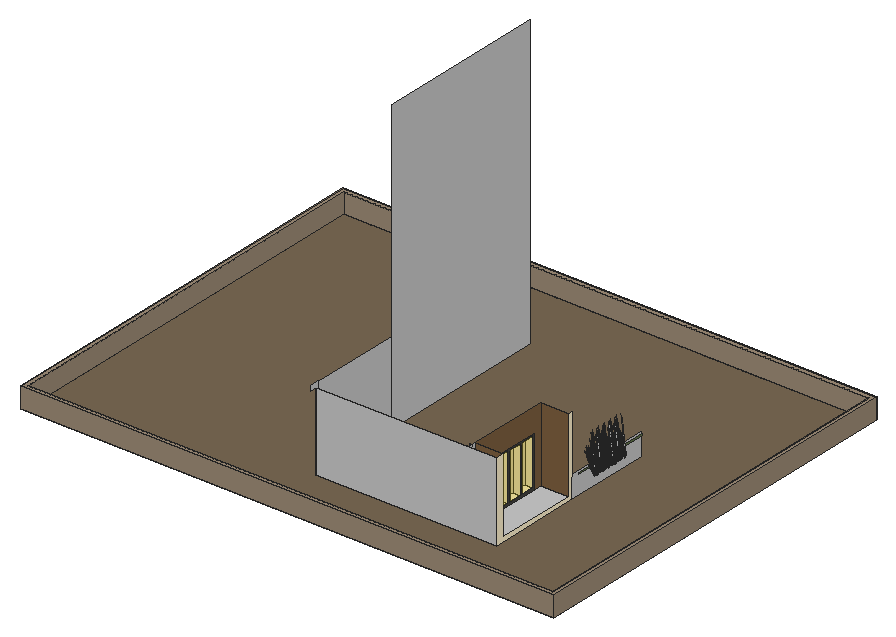
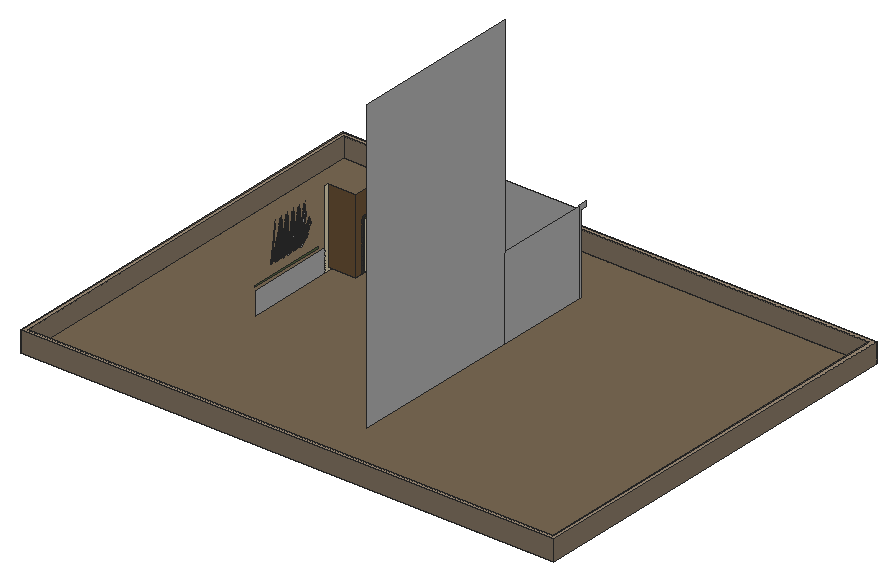
# SketchUp Ruby script. Lengths in inches.
U = 1.inch
M = Sketchup.active_model
def pt(a) = Geom::Point3d.new(a.map { |v| v * U })
def face(e, loops, mat)
  f = e.add_face(loops[0].map { |a| pt(a) })
  loops[1..].each { |l| e.add_face(l.map { |a| pt(a) }).erase! }
  f.material = f.back_material = mat if mat
  f
end
# faces: each face lists its corners as indices into pts; further lists are holes
def faces(e, pts, list, mat = nil) = list.each { |f| face(e, (f[0].is_a?(Array) ? f : [f]).map { |l| l.map { |i| pts[i] } }, mat) }
# xy, xz, yz: faces in a plane at the given z, y or x. An outline is a flat list of corners, or four numbers for a rectangle; further outlines are holes
def ring(l) = l.size == 4 ? [[l[0], l[1]], [l[2], l[1]], [l[2], l[3]], [l[0], l[3]]] : l.each_slice(2).to_a
def flat(e, list, mat, &to3) = list.each { |f| face(e, (f[0].is_a?(Array) ? f : [f]).map { |l| ring(l).map { |u, v| to3.(u, v) } }, mat) }
def xy(e, z, list, mat = nil) = flat(e, list, mat) { |x, y| [x, y, z] }
def xz(e, y, list, mat = nil) = flat(e, list, mat) { |x, z| [x, y, z] }
def yz(e, x, list, mat = nil) = flat(e, list, mat) { |y, z| [x, y, z] }
def lines(e, pts, list) = list.each { |a, b| e.add_line(pt(pts[a]), pt(pts[b])) }
# prism: a flat outline (further loops are holes) pulled along v
def prism(e, loops, v, mat = nil)
  f = face(e, loops, mat); d = Geom::Vector3d.new(v.map { |x| x * U })
  f.pushpull(f.normal.samedirection?(d) ? d.length : -d.length)
end
def box(e, o, s, mat = nil) = prism(e, [[o, [o[0] + s[0], o[1], o[2]], [o[0] + s[0], o[1] + s[1], o[2]], [o[0], o[1] + s[1], o[2]]]], [0, 0, s[2]], mat)
def at(x, y, z, deg = 0) = Geom::Transformation.translation(pt([x, y, z])) * Geom::Transformation.rotation(ORIGIN, Z_AXIS, deg.degrees)
def axes(o, x, y, z) = Geom::Transformation.new([*x, 0, *y, 0, *z, 0, *pt(o).to_a, 1])
def part(name) = M.definitions.add(name)
# library, detail: a bought-in or finely detailed component or shape, given as its bounding box
def library(name, o, s) = part(name).tap { |d| box(d.entities, o, s) }
def detail(e, o, s) = box(e.add_group.entities, o, s)
def put(e, d, t, mat = nil) = e.add_instance(d, t).tap { |i| i.material = mat if mat }
def group(e, t, mat = nil) = e.add_group.tap { |g| g.transformation = t; g.material = mat if mat }.entities
root = M.entities
M.materials.add("D01_Frost_White").color = [255, 242, 206]
M.materials.add("Glass_Basic_01").color = [255, 228, 0]
M.materials["Glass_Basic_01"].alpha = 0.25
M.materials.add("LightPink_Translucent").color = [144, 107, 117]
M.materials["LightPink_Translucent"].alpha = 0.75
M.materials.add("Plaster_02_1K").color = [157, 140, 119]
M.materials.add("Plaster_03_1K").color = [121, 105, 83]
M.materials.add("Plywood_01_1K").color = [125, 96, 64]
M.materials.add("Roofing_02_1K").color = [97, 118, 74]
M.materials.add("Tile_Exterior_08_1K").color = [62, 60, 47]
M.materials.add("Wood_Planks_01_1K").color = [69, 67, 63]
M.materials.add("[_0053_Ivory_]").color = [200, 200, 200]
c1 = part("blade")
p = [[2.15,0.21,22],[0,0.17,0],[0.09,0.45,0],[2.18,0.31,22],[2.29,0.31,22],[0.38,0.45,0],
  [2.48,0.24,33],[2.49,0.24,33],[2.48,0.22,33]]
faces(c1.entities,p,[[0,1,2,3],[4,5,2,3],[6,3,4,7],[8,0,3,6]])
c2 = part("seeds")
p = [[0.3,-0.1,1.38],[-0.01,-0.03,1.59],[-0.01,-0.03,0.03],[0.14,-0.07,-0.07],[0.29,-0.03,3],[0.15,0.01,3.11]]
faces(c2.entities,p,[[0,1,2,3],[1,0,4,5]],"LightPink_Translucent")
c3 = part("blade with seeds")
put(c3.entities,c1,at(0,0,0))
put(c3.entities,c2,axes([2.4,0.25,30.99],[1.5799,-0.05474,1.17369],[-0.12525,1.92788,0.29478],[-0.07173,-0.02425,1.56792]))
xy(root,0,[[6,6,810.43,611.69]],"Plaster_03_1K")
xy(root,0,[[[0,0,816.43,617.69],[6,6,810.43,611.69]]],"Tile_Exterior_08_1K")
xy(root,6,[[610.51,107.15,653.51,233.15]],"[_0053_Ivory_]")
xy(root,9,[[598.7,122.15,610.51,146.15],[598.51,149.15,610.51,170.15],[598.51,173.15,610.51,194.15],[598.51,197.15,610.51,218.15]],"D01_Frost_White")
xy(root,30.91,[[[0,0,816.43,617.69],[6,6,810.43,611.69]]],"Plaster_02_1K")
xz(root,0,[[0,0,816.43,30.91]],"Plaster_02_1K")
xz(root,6,[[6,0,810.43,30.91]],"Plaster_02_1K")
xz(root,94.15,[[377.51,0,653.51,120]],"[_0053_Ivory_]")
xz(root,95.51,[[607.51,6,610.51,120]],"[_0053_Ivory_]")
xz(root,101.15,[[607.51,6,610.51,120]],"[_0053_Ivory_]")
xz(root,107.15,[[610.51,6,653.51,120]],"Plywood_01_1K")
xz(root,122.15,[[598.7,9,610.51,81]],"D01_Frost_White")
xz(root,146.15,[[598.7,9,610.51,81]],"D01_Frost_White")
xz(root,149.15,[[598.51,9,610.51,81]],"D01_Frost_White")
xz(root,170.15,[[598.51,9,610.51,81]],"D01_Frost_White")
xz(root,173.15,[[598.51,9,610.51,81]],"D01_Frost_White")
xz(root,194.15,[[598.51,9,610.51,81]],"D01_Frost_White")
xz(root,197.15,[[598.51,9,610.51,81]],"D01_Frost_White")
xz(root,218.15,[[598.51,9,610.51,81]],"D01_Frost_White")
xz(root,233.15,[[610.51,6,653.51,120]],"Plywood_01_1K")
xz(root,611.69,[[6,0,810.43,30.91]],"Plaster_02_1K")
xz(root,617.69,[[0,0,816.43,30.91]],"Plaster_02_1K")
yz(root,0,[[0,0,617.69,30.91]],"Plaster_02_1K")
yz(root,6,[[6,0,611.69,30.91]],"Plaster_02_1K")
yz(root,377.51,[[94.15,0,94.15,120,83.15,120,83.15,127,98.15,127,98.15,0],[98.15,0,239.15,126],[239.15,0,503.15,444]],"[_0053_Ivory_]")
yz(root,598.51,[[149.15,9,170.15,81],[173.15,9,194.15,81],[197.15,9,218.15,81]],"D01_Frost_White")
yz(root,598.7,[[122.15,9,146.15,81]],"D01_Frost_White")
yz(root,610.51,[[122.15,9,146.15,81],[149.15,9,170.15,81],[173.15,9,194.15,81],[197.15,9,218.15,81]],"Glass_Basic_01")
yz(root,610.51,[[107.15,6,119.15,6,119.15,84,221.15,84,221.15,6,233.15,6,233.15,120,107.15,120]],"Plywood_01_1K")
yz(root,610.51,[[[119.15,6,221.15,84],[122.15,9,122.15,81,146.15,81,146.15,9,149.15,9,149.15,81,170.15,81,170.15,9,173.15,9,173.15,81,194.15,81,194.15,9,197.15,9,197.15,81,218.15,81,218.15,9]]],"Wood_Planks_01_1K")
yz(root,610.51,[[95.51,6,101.15,120],[101.15,6,107.15,120]],"[_0053_Ivory_]")
yz(root,653.51,[[94.15,0,239.15,0,239.15,120,233.15,120,233.15,6,107.15,6,107.15,120,94.15,120]],"D01_Frost_White")
yz(root,653.51,[[239.15,0,371.15,34]],"[_0053_Ivory_]")
yz(root,659.51,[[245.15,34,365.15,36]],"Roofing_02_1K")
yz(root,810.43,[[6,0,611.69,30.91]],"Plaster_02_1K")
yz(root,816.43,[[0,0,617.69,30.91]],"Plaster_02_1K")
p = [[607.51,101.15,6],[383.51,101.15,6],[383.51,95.15,6],[607.51,95.15,6],[607.51,95.51,6]]
lines(root,p,[[0,1],[2,1],[3,4]])
put(root,c3,axes([677.08,253.49,37.53],[0.25192,-0.01424,1.71376],[-0.16712,0.61729,0.13857],[-0.35901,-0.03818,0.73262]),"[_0053_Ivory_]")
put(root,c3,axes([677.08,264.64,37.53],[0.25192,-0.01424,1.71376],[-0.16712,0.61729,0.13857],[-0.35901,-0.03818,0.73262]),"[_0053_Ivory_]")
put(root,c3,axes([677.08,275.63,37.53],[0.25192,-0.01424,1.71376],[-0.16712,0.61729,0.13857],[-0.35901,-0.03818,0.73262]),"[_0053_Ivory_]")
put(root,c3,axes([677.08,287.67,37.53],[0.25192,-0.01424,1.71376],[-0.16712,0.61729,0.13857],[-0.35901,-0.03818,0.73262]),"[_0053_Ivory_]")
put(root,c3,axes([677.08,299.04,37.53],[0.25192,-0.01424,1.71376],[-0.16712,0.61729,0.13857],[-0.35901,-0.03818,0.73262]),"[_0053_Ivory_]")
put(root,c3,axes([677.08,311.02,37.53],[0.25192,-0.01424,1.71376],[-0.16712,0.61729,0.13857],[-0.35901,-0.03818,0.73262]),"[_0053_Ivory_]")
put(root,c3,axes([677.1875,254.57,37.53],[0.21074,-0.13302,1.71376],[0.17741,0.61464,0.13857],[-0.33083,0.13891,0.73262]),"[_0053_Ivory_]")
put(root,c3,axes([677.1875,265.72,37.53],[0.21074,-0.13302,1.71376],[0.17741,0.61464,0.13857],[-0.33083,0.13891,0.73262]),"[_0053_Ivory_]")
put(root,c3,axes([677.1875,276.71,37.53],[0.21074,-0.13302,1.71376],[0.17741,0.61464,0.13857],[-0.33083,0.13891,0.73262]),"[_0053_Ivory_]")
put(root,c3,axes([677.1875,288.76,37.53],[0.21074,-0.13302,1.71376],[0.17741,0.61464,0.13857],[-0.33083,0.13891,0.73262]),"[_0053_Ivory_]")
put(root,c3,axes([677.1875,300.125,37.53],[0.21074,-0.13302,1.71376],[0.17741,0.61464,0.13857],[-0.33083,0.13891,0.73262]),"[_0053_Ivory_]")
put(root,c3,axes([676.53,255.62,36.24],[0.21107,0.05162,1.43002],[0.13604,0.52729,-0.30754],[-0.28671,0.0987,0.61141]),"[_0053_Ivory_]")
put(root,c3,axes([676.53,266.77,36.24],[0.21107,0.05162,1.43002],[0.13604,0.52729,-0.30754],[-0.28671,0.0987,0.61141]),"[_0053_Ivory_]")
put(root,c3,axes([676.53,277.76,36.24],[0.21107,0.05162,1.43002],[0.13604,0.52729,-0.30754],[-0.28671,0.0987,0.61141]),"[_0053_Ivory_]")
put(root,c3,axes([676.53,289.8,36.24],[0.21107,0.05162,1.43002],[0.13604,0.52729,-0.30754],[-0.28671,0.0987,0.61141]),"[_0053_Ivory_]")
put(root,c3,axes([676.53,301.17,36.24],[0.21107,0.05162,1.43002],[0.13604,0.52729,-0.30754],[-0.28671,0.0987,0.61141]),"[_0053_Ivory_]")
put(root,c3,axes([678.4,253.93,37],[0.17264,-0.09097,1.77064],[0.05953,0.63516,0.13857],[-0.37394,0.08428,0.63284]),"[_0053_Ivory_]")
put(root,c3,axes([678.4,265.08,37],[0.17264,-0.09097,1.77064],[0.05953,0.63516,0.13857],[-0.37394,0.08428,0.63284]),"[_0053_Ivory_]")
put(root,c3,axes([678.4,276.07,37],[0.17264,-0.09097,1.77064],[0.05953,0.63516,0.13857],[-0.37394,0.08428,0.63284]),"[_0053_Ivory_]")
put(root,c3,axes([678.4,288.11,37],[0.17264,-0.09097,1.77064],[0.05953,0.63516,0.13857],[-0.37394,0.08428,0.63284]),"[_0053_Ivory_]")
put(root,c3,axes([678.4,299.48,37],[0.17264,-0.09097,1.77064],[0.05953,0.63516,0.13857],[-0.37394,0.08428,0.63284]),"[_0053_Ivory_]")
put(root,c3,axes([677.83,252.91,38.63],[-0.60713,-0.01514,-0.71045],[0.04078,-0.63759,0.08574],[-0.25721,-0.06729,1.00501]),"[_0053_Ivory_]")
put(root,c3,axes([677.83,264.0625,38.63],[-0.60713,-0.01514,-0.71045],[0.04078,-0.63759,0.08574],[-0.25721,-0.06729,1.00501]),"[_0053_Ivory_]")
put(root,c3,axes([677.83,275.05,38.63],[-0.60713,-0.01514,-0.71045],[0.04078,-0.63759,0.08574],[-0.25721,-0.06729,1.00501]),"[_0053_Ivory_]")
put(root,c3,axes([677.83,287.1,38.63],[-0.60713,-0.01514,-0.71045],[0.04078,-0.63759,0.08574],[-0.25721,-0.06729,1.00501]),"[_0053_Ivory_]")
put(root,c3,axes([677.83,298.46,38.63],[-0.60713,-0.01514,-0.71045],[0.04078,-0.63759,0.08574],[-0.25721,-0.06729,1.00501]),"[_0053_Ivory_]")
put(root,c3,axes([677.83,310.44,38.63],[-0.60713,-0.01514,-0.71045],[0.04078,-0.63759,0.08574],[-0.25721,-0.06729,1.00501]),"[_0053_Ivory_]")
put(root,c3,axes([677.35,253.07,36.24],[0.11858,0.17508,1.43002],[-0.27325,0.4759,-0.30754],[-0.28057,-0.11375,0.61141]),"[_0053_Ivory_]")
put(root,c3,axes([677.35,264.22,36.24],[0.11858,0.17508,1.43002],[-0.27325,0.4759,-0.30754],[-0.28057,-0.11375,0.61141]),"[_0053_Ivory_]")
put(root,c3,axes([677.35,275.21,36.24],[0.11858,0.17508,1.43002],[-0.27325,0.4759,-0.30754],[-0.28057,-0.11375,0.61141]),"[_0053_Ivory_]")
put(root,c3,axes([677.35,287.25,36.24],[0.11858,0.17508,1.43002],[-0.27325,0.4759,-0.30754],[-0.28057,-0.11375,0.61141]),"[_0053_Ivory_]")
put(root,c3,axes([677.35,298.62,36.24],[0.11858,0.17508,1.43002],[-0.27325,0.4759,-0.30754],[-0.28057,-0.11375,0.61141]),"[_0053_Ivory_]")
put(root,c3,axes([677.35,310.6,36.24],[0.11858,0.17508,1.43002],[-0.27325,0.4759,-0.30754],[-0.28057,-0.11375,0.61141]),"[_0053_Ivory_]")
put(root,c3,axes([676.86,254.02,38.18],[-0.50475,-0.17543,-0.35414],[0.14722,-0.5118,0.4572],[-0.20322,0.04693,0.87481]),"[_0053_Ivory_]")
put(root,c3,axes([676.86,265.17,38.18],[-0.50475,-0.17543,-0.35414],[0.14722,-0.5118,0.4572],[-0.20322,0.04693,0.87481]),"[_0053_Ivory_]")
put(root,c3,axes([676.86,276.16,38.18],[-0.50475,-0.17543,-0.35414],[0.14722,-0.5118,0.4572],[-0.20322,0.04693,0.87481]),"[_0053_Ivory_]")
put(root,c3,axes([676.86,288.2,38.18],[-0.50475,-0.17543,-0.35414],[0.14722,-0.5118,0.4572],[-0.20322,0.04693,0.87481]),"[_0053_Ivory_]")
put(root,c3,axes([676.86,299.57,38.18],[-0.50475,-0.17543,-0.35414],[0.14722,-0.5118,0.4572],[-0.20322,0.04693,0.87481]),"[_0053_Ivory_]")
put(root,c3,axes([677.56,252.5,37.53],[0.2256,0.10835,1.71376],[-0.46687,0.45453,0.13857],[-0.29098,-0.20505,0.73262]),"[_0053_Ivory_]")
put(root,c3,axes([677.56,263.64,37.53],[0.2256,0.10835,1.71376],[-0.46687,0.45453,0.13857],[-0.29098,-0.20505,0.73262]),"[_0053_Ivory_]")
put(root,c3,axes([677.56,274.64,37.53],[0.2256,0.10835,1.71376],[-0.46687,0.45453,0.13857],[-0.29098,-0.20505,0.73262]),"[_0053_Ivory_]")
put(root,c3,axes([677.56,286.68,37.53],[0.2256,0.10835,1.71376],[-0.46687,0.45453,0.13857],[-0.29098,-0.20505,0.73262]),"[_0053_Ivory_]")
put(root,c3,axes([677.56,298.05,37.53],[0.2256,0.10835,1.71376],[-0.46687,0.45453,0.13857],[-0.29098,-0.20505,0.73262]),"[_0053_Ivory_]")
put(root,c3,axes([677.56,310.02,37.53],[0.2256,0.10835,1.71376],[-0.46687,0.45453,0.13857],[-0.29098,-0.20505,0.73262]),"[_0053_Ivory_]")
put(root,c3,axes([677.21,254.28,38.33],[-0.16454,0.57202,-0.51099],[-0.56413,-0.19607,-0.3958],[-0.22713,0.05245,0.97773]),"[_0053_Ivory_]")
put(root,c3,axes([677.21,265.43,38.33],[-0.16454,0.57202,-0.51099],[-0.56413,-0.19607,-0.3958],[-0.22713,0.05245,0.97773]),"[_0053_Ivory_]")
put(root,c3,axes([677.21,276.42,38.33],[-0.16454,0.57202,-0.51099],[-0.56413,-0.19607,-0.3958],[-0.22713,0.05245,0.97773]),"[_0053_Ivory_]")
put(root,c3,axes([677.21,288.46,38.33],[-0.16454,0.57202,-0.51099],[-0.56413,-0.19607,-0.3958],[-0.22713,0.05245,0.97773]),"[_0053_Ivory_]")
put(root,c3,axes([677.21,299.83,38.33],[-0.16454,0.57202,-0.51099],[-0.56413,-0.19607,-0.3958],[-0.22713,0.05245,0.97773]),"[_0053_Ivory_]")
put(root,c3,axes([677.63,253.04,38.33],[-0.44101,0.41656,-0.51099],[-0.38623,-0.44004,-0.3958],[-0.22407,-0.06338,0.97773]),"[_0053_Ivory_]")
put(root,c3,axes([677.63,264.19,38.33],[-0.44101,0.41656,-0.51099],[-0.38623,-0.44004,-0.3958],[-0.22407,-0.06338,0.97773]),"[_0053_Ivory_]")
put(root,c3,axes([677.63,275.18,38.33],[-0.44101,0.41656,-0.51099],[-0.38623,-0.44004,-0.3958],[-0.22407,-0.06338,0.97773]),"[_0053_Ivory_]")
put(root,c3,axes([677.63,287.23,38.33],[-0.44101,0.41656,-0.51099],[-0.38623,-0.44004,-0.3958],[-0.22407,-0.06338,0.97773]),"[_0053_Ivory_]")
put(root,c3,axes([677.63,298.59,38.33],[-0.44101,0.41656,-0.51099],[-0.38623,-0.44004,-0.3958],[-0.22407,-0.06338,0.97773]),"[_0053_Ivory_]")
put(root,c3,axes([677.63,310.57,38.33],[-0.44101,0.41656,-0.51099],[-0.38623,-0.44004,-0.3958],[-0.22407,-0.06338,0.97773]),"[_0053_Ivory_]")
put(root,c3,axes([676.92,254.24,35.15],[0.0154,0.09911,1.76342],[-0.31051,0.51756,-0.26939],[-0.22056,-0.02609,0.30037]),"[_0053_Ivory_]")
put(root,c3,axes([676.92,265.39,35.15],[0.0154,0.09911,1.76342],[-0.31051,0.51756,-0.26939],[-0.22056,-0.02609,0.30037]),"[_0053_Ivory_]")
put(root,c3,axes([676.92,276.38,35.15],[0.0154,0.09911,1.76342],[-0.31051,0.51756,-0.26939],[-0.22056,-0.02609,0.30037]),"[_0053_Ivory_]")
put(root,c3,axes([676.92,288.43,35.15],[0.0154,0.09911,1.76342],[-0.31051,0.51756,-0.26939],[-0.22056,-0.02609,0.30037]),"[_0053_Ivory_]")
put(root,c3,axes([676.92,299.79,35.15],[0.0154,0.09911,1.76342],[-0.31051,0.51756,-0.26939],[-0.22056,-0.02609,0.30037]),"[_0053_Ivory_]")
put(root,c3,axes([676.09,256.73,36.42],[0.25312,-0.28501,1.1486],[0.09988,0.45119,0.84392],[-0.18292,0.08079,0.25299]),"[_0053_Ivory_]")
put(root,c3,axes([676.09,267.875,36.42],[0.25312,-0.28501,1.1486],[0.09988,0.45119,0.84392],[-0.18292,0.08079,0.25299]),"[_0053_Ivory_]")
put(root,c3,axes([676.09,278.87,36.42],[0.25312,-0.28501,1.1486],[0.09988,0.45119,0.84392],[-0.18292,0.08079,0.25299]),"[_0053_Ivory_]")
put(root,c3,axes([676.09,290.91,36.42],[0.25312,-0.28501,1.1486],[0.09988,0.45119,0.84392],[-0.18292,0.08079,0.25299]),"[_0053_Ivory_]")
put(root,c3,axes([676.09,302.28,36.42],[0.25312,-0.28501,1.1486],[0.09988,0.45119,0.84392],[-0.18292,0.08079,0.25299]),"[_0053_Ivory_]")
put(root,c3,axes([677.47,252.65,38.18],[-0.34557,-0.39372,-0.35414],[0.39459,-0.37271,0.4572],[-0.20048,-0.05671,0.87481]),"[_0053_Ivory_]")
put(root,c3,axes([677.47,263.8,38.18],[-0.34557,-0.39372,-0.35414],[0.39459,-0.37271,0.4572],[-0.20048,-0.05671,0.87481]),"[_0053_Ivory_]")
put(root,c3,axes([677.47,274.79,38.18],[-0.34557,-0.39372,-0.35414],[0.39459,-0.37271,0.4572],[-0.20048,-0.05671,0.87481]),"[_0053_Ivory_]")
put(root,c3,axes([677.47,286.83,38.18],[-0.34557,-0.39372,-0.35414],[0.39459,-0.37271,0.4572],[-0.20048,-0.05671,0.87481]),"[_0053_Ivory_]")
put(root,c3,axes([677.47,298.2,38.18],[-0.34557,-0.39372,-0.35414],[0.39459,-0.37271,0.4572],[-0.20048,-0.05671,0.87481]),"[_0053_Ivory_]")
put(root,c3,axes([677.47,310.18,38.18],[-0.34557,-0.39372,-0.35414],[0.39459,-0.37271,0.4572],[-0.20048,-0.05671,0.87481]),"[_0053_Ivory_]")
put(root,c3,axes([677.96,254.99,37.53],[0.1517,-0.19322,1.71376],[0.38303,0.52154,0.13857],[-0.26271,0.23751,0.73262]),"[_0053_Ivory_]")
put(root,c3,axes([677.96,266.14,37.53],[0.1517,-0.19322,1.71376],[0.38303,0.52154,0.13857],[-0.26271,0.23751,0.73262]),"[_0053_Ivory_]")
put(root,c3,axes([677.96,277.13,37.53],[0.1517,-0.19322,1.71376],[0.38303,0.52154,0.13857],[-0.26271,0.23751,0.73262]),"[_0053_Ivory_]")
put(root,c3,axes([677.96,289.17,37.53],[0.1517,-0.19322,1.71376],[0.38303,0.52154,0.13857],[-0.26271,0.23751,0.73262]),"[_0053_Ivory_]")
put(root,c3,axes([677.96,300.54,37.53],[0.1517,-0.19322,1.71376],[0.38303,0.52154,0.13857],[-0.26271,0.23751,0.73262]),"[_0053_Ivory_]")
put(root,c3,axes([677.04,255.49,38.18],[-0.52868,0.08987,-0.35414],[-0.1396,-0.51376,0.4572],[-0.1515,0.13799,0.87481]),"[_0053_Ivory_]")
put(root,c3,axes([677.04,266.64,38.18],[-0.52868,0.08987,-0.35414],[-0.1396,-0.51376,0.4572],[-0.1515,0.13799,0.87481]),"[_0053_Ivory_]")
put(root,c3,axes([677.04,277.63,38.18],[-0.52868,0.08987,-0.35414],[-0.1396,-0.51376,0.4572],[-0.1515,0.13799,0.87481]),"[_0053_Ivory_]")
put(root,c3,axes([677.04,289.68,38.18],[-0.52868,0.08987,-0.35414],[-0.1396,-0.51376,0.4572],[-0.1515,0.13799,0.87481]),"[_0053_Ivory_]")
put(root,c3,axes([677.04,301.04,38.18],[-0.52868,0.08987,-0.35414],[-0.1396,-0.51376,0.4572],[-0.1515,0.13799,0.87481]),"[_0053_Ivory_]")
put(root,c3,axes([676.76,257.02,35.15],[0.08147,0.06283,1.76342],[0.13814,0.58211,-0.26939],[-0.18056,0.12413,0.30037]),"[_0053_Ivory_]")
put(root,c3,axes([676.76,268.17,35.15],[0.08147,0.06283,1.76342],[0.13814,0.58211,-0.26939],[-0.18056,0.12413,0.30037]),"[_0053_Ivory_]")
put(root,c3,axes([676.76,279.16,35.15],[0.08147,0.06283,1.76342],[0.13814,0.58211,-0.26939],[-0.18056,0.12413,0.30037]),"[_0053_Ivory_]")
put(root,c3,axes([676.76,291.2,35.15],[0.08147,0.06283,1.76342],[0.13814,0.58211,-0.26939],[-0.18056,0.12413,0.30037]),"[_0053_Ivory_]")
put(root,c3,axes([676.76,302.57,35.15],[0.08147,0.06283,1.76342],[0.13814,0.58211,-0.26939],[-0.18056,0.12413,0.30037]),"[_0053_Ivory_]")
put(root,c3,axes([676.64,253.59,36.42],[0.38775,-0.045,1.1486],[-0.24596,0.39648,0.84392],[-0.19161,-0.05948,0.25299]),"[_0053_Ivory_]")
put(root,c3,axes([676.64,264.74,36.42],[0.38775,-0.045,1.1486],[-0.24596,0.39648,0.84392],[-0.19161,-0.05948,0.25299]),"[_0053_Ivory_]")
put(root,c3,axes([676.64,275.73,36.42],[0.38775,-0.045,1.1486],[-0.24596,0.39648,0.84392],[-0.19161,-0.05948,0.25299]),"[_0053_Ivory_]")
put(root,c3,axes([676.64,287.78,36.42],[0.38775,-0.045,1.1486],[-0.24596,0.39648,0.84392],[-0.19161,-0.05948,0.25299]),"[_0053_Ivory_]")
put(root,c3,axes([676.64,299.15,36.42],[0.38775,-0.045,1.1486],[-0.24596,0.39648,0.84392],[-0.19161,-0.05948,0.25299]),"[_0053_Ivory_]")
put(root,c3,axes([676.64,311.12,36.42],[0.38775,-0.045,1.1486],[-0.24596,0.39648,0.84392],[-0.19161,-0.05948,0.25299]),"[_0053_Ivory_]")
put(root,c3,axes([677.84,255.46,37.53],[0.11309,-0.21615,1.71376],[0.47441,0.44731,0.13857],[-0.21402,0.27879,0.73262]),"[_0053_Ivory_]")
put(root,c3,axes([677.84,266.61,37.53],[0.11309,-0.21615,1.71376],[0.47441,0.44731,0.13857],[-0.21402,0.27879,0.73262]),"[_0053_Ivory_]")
put(root,c3,axes([677.84,277.6,37.53],[0.11309,-0.21615,1.71376],[0.47441,0.44731,0.13857],[-0.21402,0.27879,0.73262]),"[_0053_Ivory_]")
put(root,c3,axes([677.84,289.65,37.53],[0.11309,-0.21615,1.71376],[0.47441,0.44731,0.13857],[-0.21402,0.27879,0.73262]),"[_0053_Ivory_]")
put(root,c3,axes([677.84,301.01,37.53],[0.11309,-0.21615,1.71376],[0.47441,0.44731,0.13857],[-0.21402,0.27879,0.73262]),"[_0053_Ivory_]")
put(root,c3,axes([677.48,255.55,38.33],[0.15602,0.5742,-0.51099],[-0.59087,0.10045,-0.3958],[-0.16933,0.15423,0.97773]),"[_0053_Ivory_]")
put(root,c3,axes([677.48,266.7,38.33],[0.15602,0.5742,-0.51099],[-0.59087,0.10045,-0.3958],[-0.16933,0.15423,0.97773]),"[_0053_Ivory_]")
put(root,c3,axes([677.48,277.69,38.33],[0.15602,0.5742,-0.51099],[-0.59087,0.10045,-0.3958],[-0.16933,0.15423,0.97773]),"[_0053_Ivory_]")
put(root,c3,axes([677.48,289.74,38.33],[0.15602,0.5742,-0.51099],[-0.59087,0.10045,-0.3958],[-0.16933,0.15423,0.97773]),"[_0053_Ivory_]")
put(root,c3,axes([677.48,301.1,38.33],[0.15602,0.5742,-0.51099],[-0.59087,0.10045,-0.3958],[-0.16933,0.15423,0.97773]),"[_0053_Ivory_]")
put(root,c3,axes([678.95,255.14,35.71],[-0.63179,-0.1031,-0.62353],[0.13332,-0.63596,-0.16365],[-0.18854,-0.07706,1.37633]),"[_0053_Ivory_]")
put(root,c3,axes([678.95,266.29,35.71],[-0.63179,-0.1031,-0.62353],[0.13332,-0.63596,-0.16365],[-0.18854,-0.07706,1.37633]),"[_0053_Ivory_]")
put(root,c3,axes([678.95,277.28,35.71],[-0.63179,-0.1031,-0.62353],[0.13332,-0.63596,-0.16365],[-0.18854,-0.07706,1.37633]),"[_0053_Ivory_]")
put(root,c3,axes([678.95,289.32,35.71],[-0.63179,-0.1031,-0.62353],[0.13332,-0.63596,-0.16365],[-0.18854,-0.07706,1.37633]),"[_0053_Ivory_]")
put(root,c3,axes([678.95,300.69,35.71],[-0.63179,-0.1031,-0.62353],[0.13332,-0.63596,-0.16365],[-0.18854,-0.07706,1.37633]),"[_0053_Ivory_]")
put(root,c3,axes([678.89,252.16,38.63],[-0.51789,-0.30395,-0.71045],[0.36805,-0.53263,0.08574],[-0.18764,-0.18149,1.00501]),"[_0053_Ivory_]")
put(root,c3,axes([678.89,263.3125,38.63],[-0.51789,-0.30395,-0.71045],[0.36805,-0.53263,0.08574],[-0.18764,-0.18149,1.00501]),"[_0053_Ivory_]")
put(root,c3,axes([678.89,274.3,38.63],[-0.51789,-0.30395,-0.71045],[0.36805,-0.53263,0.08574],[-0.18764,-0.18149,1.00501]),"[_0053_Ivory_]")
put(root,c3,axes([678.89,286.35,38.63],[-0.51789,-0.30395,-0.71045],[0.36805,-0.53263,0.08574],[-0.18764,-0.18149,1.00501]),"[_0053_Ivory_]")
put(root,c3,axes([678.89,297.71,38.63],[-0.51789,-0.30395,-0.71045],[0.36805,-0.53263,0.08574],[-0.18764,-0.18149,1.00501]),"[_0053_Ivory_]")
put(root,c3,axes([678.89,309.69,38.63],[-0.51789,-0.30395,-0.71045],[0.36805,-0.53263,0.08574],[-0.18764,-0.18149,1.00501]),"[_0053_Ivory_]")
put(root,c3,axes([678.65,252.18,38.33],[-0.59932,0.14948,-0.51099],[-0.10484,-0.56611,-0.3958],[-0.16097,-0.16223,0.97773]),"[_0053_Ivory_]")
put(root,c3,axes([678.65,263.33,38.33],[-0.59932,0.14948,-0.51099],[-0.10484,-0.56611,-0.3958],[-0.16097,-0.16223,0.97773]),"[_0053_Ivory_]")
put(root,c3,axes([678.65,274.32,38.33],[-0.59932,0.14948,-0.51099],[-0.10484,-0.56611,-0.3958],[-0.16097,-0.16223,0.97773]),"[_0053_Ivory_]")
put(root,c3,axes([678.65,286.36,38.33],[-0.59932,0.14948,-0.51099],[-0.10484,-0.56611,-0.3958],[-0.16097,-0.16223,0.97773]),"[_0053_Ivory_]")
put(root,c3,axes([678.65,297.73,38.33],[-0.59932,0.14948,-0.51099],[-0.10484,-0.56611,-0.3958],[-0.16097,-0.16223,0.97773]),"[_0053_Ivory_]")
put(root,c3,axes([678.65,309.71,38.33],[-0.59932,0.14948,-0.51099],[-0.10484,-0.56611,-0.3958],[-0.16097,-0.16223,0.97773]),"[_0053_Ivory_]")
put(root,c3,axes([678.125,256.34,35.67],[-0.56842,-0.31443,-0.49651],[0.33976,-0.56381,0],[-0.12946,-0.07161,1.57504]),"[_0053_Ivory_]")
put(root,c3,axes([678.125,267.49,35.67],[-0.56842,-0.31443,-0.49651],[0.33976,-0.56381,0],[-0.12946,-0.07161,1.57504]),"[_0053_Ivory_]")
put(root,c3,axes([678.125,278.48,35.67],[-0.56842,-0.31443,-0.49651],[0.33976,-0.56381,0],[-0.12946,-0.07161,1.57504]),"[_0053_Ivory_]")
put(root,c3,axes([678.125,290.53,35.67],[-0.56842,-0.31443,-0.49651],[0.33976,-0.56381,0],[-0.12946,-0.07161,1.57504]),"[_0053_Ivory_]")
put(root,c3,axes([678.125,301.9,35.67],[-0.56842,-0.31443,-0.49651],[0.33976,-0.56381,0],[-0.12946,-0.07161,1.57504]),"[_0053_Ivory_]")
put(root,c3,axes([677.875,251.66,35.15],[-0.05883,0.08284,1.76342],[-0.59454,0.17861,-0.26939],[-0.14363,-0.16248,0.30037]),"[_0053_Ivory_]")
put(root,c3,axes([677.875,262.81,35.15],[-0.05883,0.08284,1.76342],[-0.59454,0.17861,-0.26939],[-0.14363,-0.16248,0.30037]),"[_0053_Ivory_]")
put(root,c3,axes([677.875,273.8,35.15],[-0.05883,0.08284,1.76342],[-0.59454,0.17861,-0.26939],[-0.14363,-0.16248,0.30037]),"[_0053_Ivory_]")
put(root,c3,axes([677.875,285.84,35.15],[-0.05883,0.08284,1.76342],[-0.59454,0.17861,-0.26939],[-0.14363,-0.16248,0.30037]),"[_0053_Ivory_]")
put(root,c3,axes([677.875,297.21,35.15],[-0.05883,0.08284,1.76342],[-0.59454,0.17861,-0.26939],[-0.14363,-0.16248,0.30037]),"[_0053_Ivory_]")
put(root,c3,axes([677.875,309.19,35.15],[-0.05883,0.08284,1.76342],[-0.59454,0.17861,-0.26939],[-0.14363,-0.16248,0.30037]),"[_0053_Ivory_]")
put(root,c3,axes([678.47,256.72,36.03],[-0.37973,0.63014,0],[-0.6353,-0.35142,-0.51607],[-0.14469,-0.08004,1.63711]),"[_0053_Ivory_]")
put(root,c3,axes([678.47,267.87,36.03],[-0.37973,0.63014,0],[-0.6353,-0.35142,-0.51607],[-0.14469,-0.08004,1.63711]),"[_0053_Ivory_]")
put(root,c3,axes([678.47,278.86,36.03],[-0.37973,0.63014,0],[-0.6353,-0.35142,-0.51607],[-0.14469,-0.08004,1.63711]),"[_0053_Ivory_]")
put(root,c3,axes([678.47,290.91,36.03],[-0.37973,0.63014,0],[-0.6353,-0.35142,-0.51607],[-0.14469,-0.08004,1.63711]),"[_0053_Ivory_]")
put(root,c3,axes([678.47,302.28,36.03],[-0.37973,0.63014,0],[-0.6353,-0.35142,-0.51607],[-0.14469,-0.08004,1.63711]),"[_0053_Ivory_]")
put(root,c3,axes([677.78,257.64,36.24],[0.19166,-0.0992,1.43002],[0.4732,0.29912,-0.30754],[-0.14084,0.25882,0.61141]),"[_0053_Ivory_]")
put(root,c3,axes([677.78,268.79,36.24],[0.19166,-0.0992,1.43002],[0.4732,0.29912,-0.30754],[-0.14084,0.25882,0.61141]),"[_0053_Ivory_]")
put(root,c3,axes([677.78,279.78,36.24],[0.19166,-0.0992,1.43002],[0.4732,0.29912,-0.30754],[-0.14084,0.25882,0.61141]),"[_0053_Ivory_]")
put(root,c3,axes([677.78,291.82,36.24],[0.19166,-0.0992,1.43002],[0.4732,0.29912,-0.30754],[-0.14084,0.25882,0.61141]),"[_0053_Ivory_]")
put(root,c3,axes([677.78,303.1875,36.24],[0.19166,-0.0992,1.43002],[0.4732,0.29912,-0.30754],[-0.14084,0.25882,0.61141]),"[_0053_Ivory_]")
put(root,c3,axes([677.51,251.98,35.78],[-0.1752,0.51349,-0.03893],[-0.53924,-0.15795,-0.17649],[-0.08187,-0.08399,0.58215]),"[_0053_Ivory_]")
put(root,c3,axes([677.51,263.13,35.78],[-0.1752,0.51349,-0.03893],[-0.53924,-0.15795,-0.17649],[-0.08187,-0.08399,0.58215]),"[_0053_Ivory_]")
put(root,c3,axes([677.51,274.12,35.78],[-0.1752,0.51349,-0.03893],[-0.53924,-0.15795,-0.17649],[-0.08187,-0.08399,0.58215]),"[_0053_Ivory_]")
put(root,c3,axes([677.51,286.16,35.78],[-0.1752,0.51349,-0.03893],[-0.53924,-0.15795,-0.17649],[-0.08187,-0.08399,0.58215]),"[_0053_Ivory_]")
put(root,c3,axes([677.51,297.53,35.78],[-0.1752,0.51349,-0.03893],[-0.53924,-0.15795,-0.17649],[-0.08187,-0.08399,0.58215]),"[_0053_Ivory_]")
put(root,c3,axes([677.51,309.51,35.78],[-0.1752,0.51349,-0.03893],[-0.53924,-0.15795,-0.17649],[-0.08187,-0.08399,0.58215]),"[_0053_Ivory_]")
put(root,c3,axes([678.3125,251.33,36.24],[-0.03678,0.20572,1.43002],[-0.53767,0.17221,-0.30754],[-0.12568,-0.26589,0.61141]),"[_0053_Ivory_]")
put(root,c3,axes([678.3125,262.48,36.24],[-0.03678,0.20572,1.43002],[-0.53767,0.17221,-0.30754],[-0.12568,-0.26589,0.61141]),"[_0053_Ivory_]")
put(root,c3,axes([678.3125,273.47,36.24],[-0.03678,0.20572,1.43002],[-0.53767,0.17221,-0.30754],[-0.12568,-0.26589,0.61141]),"[_0053_Ivory_]")
put(root,c3,axes([678.3125,285.52,36.24],[-0.03678,0.20572,1.43002],[-0.53767,0.17221,-0.30754],[-0.12568,-0.26589,0.61141]),"[_0053_Ivory_]")
put(root,c3,axes([678.3125,296.88,36.24],[-0.03678,0.20572,1.43002],[-0.53767,0.17221,-0.30754],[-0.12568,-0.26589,0.61141]),"[_0053_Ivory_]")
put(root,c3,axes([678.3125,308.86,36.24],[-0.03678,0.20572,1.43002],[-0.53767,0.17221,-0.30754],[-0.12568,-0.26589,0.61141]),"[_0053_Ivory_]")
put(root,c3,axes([678.49,251.87,37.53],[0.13883,0.2019,1.71376],[-0.64153,0.16998,0.13857],[-0.14499,-0.31697,0.73262]),"[_0053_Ivory_]")
put(root,c3,axes([678.49,263.01,37.53],[0.13883,0.2019,1.71376],[-0.64153,0.16998,0.13857],[-0.14499,-0.31697,0.73262]),"[_0053_Ivory_]")
put(root,c3,axes([678.49,274.01,37.53],[0.13883,0.2019,1.71376],[-0.64153,0.16998,0.13857],[-0.14499,-0.31697,0.73262]),"[_0053_Ivory_]")
put(root,c3,axes([678.49,286.05,37.53],[0.13883,0.2019,1.71376],[-0.64153,0.16998,0.13857],[-0.14499,-0.31697,0.73262]),"[_0053_Ivory_]")
put(root,c3,axes([678.49,297.42,37.53],[0.13883,0.2019,1.71376],[-0.64153,0.16998,0.13857],[-0.14499,-0.31697,0.73262]),"[_0053_Ivory_]")
put(root,c3,axes([678.49,309.39,37.53],[0.13883,0.2019,1.71376],[-0.64153,0.16998,0.13857],[-0.14499,-0.31697,0.73262]),"[_0053_Ivory_]")
put(root,c3,axes([679.67,255.24,36.32],[-0.61322,0.4175,-0.29095],[-0.40778,-0.58992,-0.50002],[-0.1513,-0.05991,1.59708]),"[_0053_Ivory_]")
put(root,c3,axes([679.67,266.38,36.32],[-0.61322,0.4175,-0.29095],[-0.40778,-0.58992,-0.50002],[-0.1513,-0.05991,1.59708]),"[_0053_Ivory_]")
put(root,c3,axes([679.67,277.375,36.32],[-0.61322,0.4175,-0.29095],[-0.40778,-0.58992,-0.50002],[-0.1513,-0.05991,1.59708]),"[_0053_Ivory_]")
put(root,c3,axes([679.67,289.42,36.32],[-0.61322,0.4175,-0.29095],[-0.40778,-0.58992,-0.50002],[-0.1513,-0.05991,1.59708]),"[_0053_Ivory_]")
put(root,c3,axes([679.67,300.79,36.32],[-0.61322,0.4175,-0.29095],[-0.40778,-0.58992,-0.50002],[-0.1513,-0.05991,1.59708]),"[_0053_Ivory_]")
put(root,c3,axes([678.71,251.76,38.18],[-0.0938,-0.50652,-0.35414],[0.53623,-0.13375,0.4572],[-0.14403,-0.14515,0.87481]),"[_0053_Ivory_]")
put(root,c3,axes([678.71,262.91,38.18],[-0.0938,-0.50652,-0.35414],[0.53623,-0.13375,0.4572],[-0.14403,-0.14515,0.87481]),"[_0053_Ivory_]")
put(root,c3,axes([678.71,273.9,38.18],[-0.0938,-0.50652,-0.35414],[0.53623,-0.13375,0.4572],[-0.14403,-0.14515,0.87481]),"[_0053_Ivory_]")
put(root,c3,axes([678.71,285.94,38.18],[-0.0938,-0.50652,-0.35414],[0.53623,-0.13375,0.4572],[-0.14403,-0.14515,0.87481]),"[_0053_Ivory_]")
put(root,c3,axes([678.71,297.3125,38.18],[-0.0938,-0.50652,-0.35414],[0.53623,-0.13375,0.4572],[-0.14403,-0.14515,0.87481]),"[_0053_Ivory_]")
put(root,c3,axes([678.71,309.29,38.18],[-0.0938,-0.50652,-0.35414],[0.53623,-0.13375,0.4572],[-0.14403,-0.14515,0.87481]),"[_0053_Ivory_]")
put(root,c3,axes([677.22,254.32,36.03],[-0.75945,0,0],[0,-0.70283,-0.51607],[0,-0.16007,1.63711]),"[_0053_Ivory_]")
put(root,c3,axes([677.22,265.47,36.03],[-0.75945,0,0],[0,-0.70283,-0.51607],[0,-0.16007,1.63711]),"[_0053_Ivory_]")
put(root,c3,axes([677.22,276.46,36.03],[-0.75945,0,0],[0,-0.70283,-0.51607],[0,-0.16007,1.63711]),"[_0053_Ivory_]")
put(root,c3,axes([677.22,288.51,36.03],[-0.75945,0,0],[0,-0.70283,-0.51607],[0,-0.16007,1.63711]),"[_0053_Ivory_]")
put(root,c3,axes([677.22,299.875,36.03],[-0.75945,0,0],[0,-0.70283,-0.51607],[0,-0.16007,1.63711]),"[_0053_Ivory_]")
put(root,c3,axes([677.22,311.85,36.03],[-0.75945,0,0],[0,-0.70283,-0.51607],[0,-0.16007,1.63711]),"[_0053_Ivory_]")
put(root,c3,axes([678.28,256.11,35.68],[-0.14267,-0.54795,-0.30978],[0.56663,-0.1556,0.30978],[-0.11423,-0.06319,1.38974]),"[_0053_Ivory_]")
put(root,c3,axes([678.28,267.26,35.68],[-0.14267,-0.54795,-0.30978],[0.56663,-0.1556,0.30978],[-0.11423,-0.06319,1.38974]),"[_0053_Ivory_]")
put(root,c3,axes([678.28,278.25,35.68],[-0.14267,-0.54795,-0.30978],[0.56663,-0.1556,0.30978],[-0.11423,-0.06319,1.38974]),"[_0053_Ivory_]")
put(root,c3,axes([678.28,290.29,35.68],[-0.14267,-0.54795,-0.30978],[0.56663,-0.1556,0.30978],[-0.11423,-0.06319,1.38974]),"[_0053_Ivory_]")
put(root,c3,axes([678.28,301.66,35.68],[-0.14267,-0.54795,-0.30978],[0.56663,-0.1556,0.30978],[-0.11423,-0.06319,1.38974]),"[_0053_Ivory_]")
